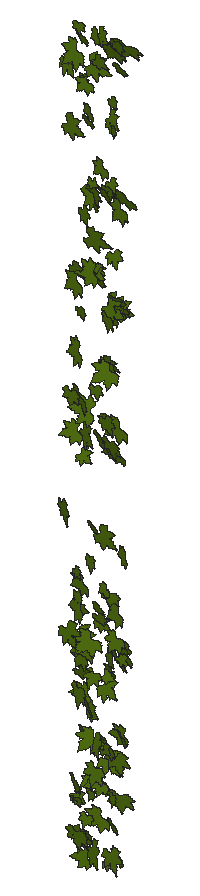
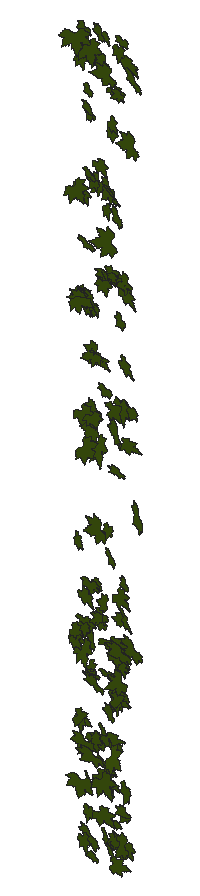
# SketchUp Ruby script. Lengths in inches.
U = 1.inch
M = Sketchup.active_model
def pt(a) = Geom::Point3d.new(a.map { |v| v * U })
def face(e, loops, mat)
  f = e.add_face(loops[0].map { |a| pt(a) })
  loops[1..].each { |l| e.add_face(l.map { |a| pt(a) }).erase! }
  f.material = f.back_material = mat if mat
  f
end
# faces: each face lists its corners as indices into pts; further lists are holes
def faces(e, pts, list, mat = nil) = list.each { |f| face(e, (f[0].is_a?(Array) ? f : [f]).map { |l| l.map { |i| pts[i] } }, mat) }
# xy, xz, yz: faces in a plane at the given z, y or x. An outline is a flat list of corners, or four numbers for a rectangle; further outlines are holes
def ring(l) = l.size == 4 ? [[l[0], l[1]], [l[2], l[1]], [l[2], l[3]], [l[0], l[3]]] : l.each_slice(2).to_a
def flat(e, list, mat, &to3) = list.each { |f| face(e, (f[0].is_a?(Array) ? f : [f]).map { |l| ring(l).map { |u, v| to3.(u, v) } }, mat) }
def xy(e, z, list, mat = nil) = flat(e, list, mat) { |x, y| [x, y, z] }
def xz(e, y, list, mat = nil) = flat(e, list, mat) { |x, z| [x, y, z] }
def yz(e, x, list, mat = nil) = flat(e, list, mat) { |y, z| [x, y, z] }
def lines(e, pts, list) = list.each { |a, b| e.add_line(pt(pts[a]), pt(pts[b])) }
# prism: a flat outline (further loops are holes) pulled along v
def prism(e, loops, v, mat = nil)
  f = face(e, loops, mat); d = Geom::Vector3d.new(v.map { |x| x * U })
  f.pushpull(f.normal.samedirection?(d) ? d.length : -d.length)
end
def box(e, o, s, mat = nil) = prism(e, [[o, [o[0] + s[0], o[1], o[2]], [o[0] + s[0], o[1] + s[1], o[2]], [o[0], o[1] + s[1], o[2]]]], [0, 0, s[2]], mat)
def at(x, y, z, deg = 0) = Geom::Transformation.translation(pt([x, y, z])) * Geom::Transformation.rotation(ORIGIN, Z_AXIS, deg.degrees)
def axes(o, x, y, z) = Geom::Transformation.new([*x, 0, *y, 0, *z, 0, *pt(o).to_a, 1])
def part(name) = M.definitions.add(name)
# library, detail: a bought-in or finely detailed component or shape, given as its bounding box
def library(name, o, s) = part(name).tap { |d| box(d.entities, o, s) }
def detail(e, o, s) = box(e.add_group.entities, o, s)
def put(e, d, t, mat = nil) = e.add_instance(d, t).tap { |i| i.material = mat if mat }
def group(e, t, mat = nil) = e.add_group.tap { |g| g.transformation = t; g.material = mat if mat }.entities
root = M.entities
M.materials.add("[Vegetation Blur 03]").color = [83, 114, 18]
c1 = part("ivy")
xy(c1.entities,0,[[0.782,0,0.786,0,0.787,0.005,0.789,0.009,0.821,0.072,0.875,0.147,1.001,0.272,1.073,0.331,1.137,0.363,1.178,0.379,1.223,0.384,1.272,0.383,1.311,0.374,1.36,0.355,1.399,0.334,1.491,0.285,1.541,0.244,1.583,0.199,1.617,0.15,1.64,0.128,1.662,0.115,1.717,0.105,1.745,0.093,1.784,0.054,1.819,0.057,1.854,0.064,1.882,0.075,1.896,0.074,1.91,0.071,1.937,0.063,1.964,0.053,1.99,0.038,2.016,0.015,2.034,0.002,2.04,0,2.038,0.003,2.036,0.007,2.033,0.038,2.036,0.068,2.045,0.1,2.055,0.116,2.064,0.123,2.077,0.129,2.088,0.129,2.106,0.132,2.118,0.13,2.179,0.132,2.207,0.133,2.225,0.133,2.242,0.138,2.22,0.162,2.207,0.186,2.206,0.213,2.212,0.236,2.228,0.262,2.247,0.274,2.298,0.283,2.355,0.294,2.37,0.296,2.376,0.295,2.377,0.3,2.377,0.303,2.385,0.329,2.411,0.37,2.426,0.392,2.449,0.407,2.511,0.426,2.561,0.444,2.619,0.466,2.589,0.469,2.561,0.476,2.501,0.5,2.449,0.516,2.424,0.523,2.401,0.535,2.377,0.556,2.372,0.568,2.36,0.575,2.268,0.586,2.225,0.592,2.207,0.599,2.194,0.61,2.143,0.65,2.13,0.664,2.122,0.682,2.123,0.7,2.13,0.719,2.148,0.75,2.17,0.781,2.195,0.807,2.221,0.828,2.284,0.874,2.291,0.88,2.288,0.887,2.276,0.9,2.267,0.916,2.265,0.933,2.273,0.967,2.292,1.002,2.313,1.03,2.334,1.054,2.348,1.067,2.358,1.074,2.363,1.076,2.362,1.081,2.35,1.094,2.347,1.11,2.35,1.143,2.359,1.18,2.385,1.254,2.415,1.324,2.448,1.393,2.45,1.4,2.446,1.398,2.44,1.394,2.427,1.383,2.402,1.36,2.376,1.339,2.345,1.324,2.305,1.309,2.282,1.303,2.273,1.306,2.245,1.294,2.212,1.287,2.187,1.291,2.163,1.301,2.142,1.316,2.134,1.327,2.124,1.325,2.09,1.292,2.053,1.259,2.014,1.234,1.973,1.215,1.954,1.21,1.931,1.208,1.909,1.212,1.893,1.22,1.879,1.233,1.872,1.248,1.867,1.281,1.864,1.319,1.821,1.258,1.773,1.197,1.726,1.141,1.698,1.121,1.679,1.116,1.666,1.117,1.647,1.122,1.632,1.129,1.62,1.141,1.617,1.154,1.617,1.219,1.621,1.254,1.623,1.268,1.623,1.281,1.618,1.314,1.606,1.346,1.603,1.375,1.607,1.403,1.603,1.467,1.599,1.499,1.605,1.525,1.614,1.552,1.629,1.577,1.635,1.589,1.629,1.587,1.618,1.582,1.596,1.566,1.581,1.556,1.568,1.552,1.557,1.55,1.545,1.553,1.531,1.562,1.522,1.572,1.504,1.591,1.486,1.611,1.474,1.631,1.457,1.666,1.455,1.684,1.457,1.698,1.452,1.715,1.444,1.728,1.424,1.754,1.419,1.772,1.423,1.786,1.434,1.819,1.444,1.848,1.446,1.855,1.44,1.861,1.43,1.867,1.386,1.904,1.349,1.948,1.326,1.973,1.31,1.995,1.288,2.048,1.284,2.153,1.287,2.254,1.284,2.255,1.282,2.253,1.278,2.247,1.274,2.237,1.266,2.216,1.226,2.125,1.208,2.076,1.184,2.033,1.155,1.984,1.135,1.942,1.111,1.899,1.083,1.861,1.053,1.85,1.059,1.83,1.061,1.809,1.056,1.79,1.049,1.767,1.04,1.749,1.018,1.733,0.994,1.726,0.942,1.734,0.95,1.6875,0.944,1.645,0.932,1.608,0.911,1.585,0.881,1.58,0.854,1.582,0.828,1.588,0.785,1.618,0.773,1.625,0.775,1.614,0.779,1.598,0.796,1.502,0.818,1.402,0.861,1.283,0.882,1.224,0.894,1.174,0.892,1.148,0.886,1.123,0.881,1.107,0.872,1.099,0.849,1.094,0.818,1.092,0.789,1.098,0.762,1.107,0.753,1.113,0.721,1.139,0.698,1.163,0.678,1.194,0.665,1.224,0.628,1.28,0.612,1.312,0.606,1.327,0.606,1.314,0.599,1.282,0.594,1.267,0.581,1.256,0.544,1.245,0.512,1.244,0.473,1.249,0.444,1.256,0.382,1.288,0.339,1.306,0.324,1.316,0.317,1.324,0.309,1.326,0.27,1.314,0.227,1.313,0.185,1.3125,0.152,1.317,0.122,1.328,0.092,1.345,0.073,1.353,0.079,1.338,0.092,1.308,0.117,1.249,0.13,1.215,0.139,1.164,0.147,1.148,0.157,1.136,0.163,1.122,0.174,1.086,0.177,1.067,0.182,1.054,0.186,1.043,0.191,1.038,0.211,1.028,0.237,1.005,0.25,0.974,0.253,0.96,0.25,0.944,0.242,0.914,0.243,0.906,0.249,0.902,0.26,0.894,0.289,0.88,0.307,0.873,0.322,0.862,0.364,0.799,0.403,0.738,0.431,0.709,0.439,0.691,0.441,0.678,0.4375,0.66,0.428,0.645,0.394,0.623,0.303,0.594,0.255,0.581,0.214,0.577,0.179,0.573,0.173,0.568,0.175,0.561,0.167,0.55,0.141,0.523,0.113,0.503,0.077,0.49,0.045,0.486,0.026,0.485,0.019,0.486,0.011,0.483,0,0.471,0.014,0.467,0.044,0.455,0.058,0.447,0.07,0.438,0.097,0.411,0.125,0.394,0.158,0.377,0.174,0.366,0.182,0.359,0.185,0.361,0.242,0.331,0.253,0.316,0.258,0.303,0.262,0.283,0.274,0.278,0.308,0.274,0.341,0.252,0.366,0.226,0.366,0.222,0.37,0.22,0.38,0.221,0.395,0.221,0.425,0.216,0.45,0.207,0.465,0.192,0.473,0.178,0.484,0.15,0.489,0.116,0.483,0.089,0.468,0.058,0.45,0.035,0.435,0.018,0.429,0.011,0.434,0.012,0.438,0.014,0.469,0.019,0.542,0.016,0.581,0.015,0.612,0.027,0.68,0.055,0.696,0.057,0.712,0.052,0.73,0.045,0.741,0.036,0.766,0.014]])
put(root,c1,axes([70.27,173.7,76.7],[0.25465,-0.11048,-0.36792],[-0.45313,-0.12762,-0.20287],[0.02807,-1.05778,0.0629]),"[Vegetation Blur 03]")
put(root,c1,axes([69.17,173.7,94.66],[0.3032,0.00804,0.42723],[0.50376,-0.343,-0.23711],[-0.14236,-1.19666,0.07083]),"[Vegetation Blur 03]")
put(root,c1,axes([69.13,173.7,72.18],[0.48124,-0.36893,0.30519],[0.35516,-0.24188,-0.41903],[-0.21409,-1.23057,-0.00913]),"[Vegetation Blur 03]")
put(root,c1,axes([69.06,173.7,65.4375],[0.45366,-0.05419,0.38117],[0.46073,-0.18,-0.36926],[-0.08098,-1.3277,0.0345]),"[Vegetation Blur 03]")
put(root,c1,axes([69.46,173.7,78.17],[0.49069,-0.15556,0.05335],[0.06086,-0.06942,-0.40473],[-0.07927,-1.0163,0.01948]),"[Vegetation Blur 03]")
put(root,c1,axes([70.36,173.7,80.93],[0.29092,-0.24551,-0.40873],[-0.49509,0.19114,-0.25278],[-0.14116,-1.1764,0.04423]),"[Vegetation Blur 03]")
put(root,c1,axes([70.1,173.7,84.52],[0.43677,-0.25618,-0.34823],[-0.42807,0.08886,-0.36791],[-0.11962,-1.25334,0.04509]),"[Vegetation Blur 03]")
put(root,c1,axes([70.52,173.7,67.91],[0.26701,-0.30376,-0.4486],[-0.53833,0.27065,-0.24226],[-0.1847,-1.22801,0.05757]),"[Vegetation Blur 03]")
put(root,c1,axes([69.35,173.7,91.19],[0.18628,-0.03587,0.49266],[0.60208,-0.08964,-0.15266],[-0.04677,-1.29689,-0.00307]),"[Vegetation Blur 03]")
put(root,c1,axes([70.78,173.7,60.76],[0.09506,0.21771,-0.46057],[-0.55663,0.32363,-0.05246],[-0.14082,-1.13231,-0.10355]),"[Vegetation Blur 03]")
put(root,c1,axes([70.41,173.7,68.89],[0.30205,-0.06223,-0.36549],[-0.44449,0.11303,-0.2477],[-0.06243,-1.1058,-0.00475]),"[Vegetation Blur 03]")
put(root,c1,axes([69.84,173.7,57.14],[0.28399,-0.06546,0.07539],[0.09562,0.06624,-0.23087],[-0.02006,-0.61097,-0.03311]),"[Vegetation Blur 03]")
put(root,c1,axes([70.01,173.7,96.4],[0.54958,-0.28156,-0.28314],[-0.3622,-0.10008,-0.45262],[-0.08884,-1.33367,0.09374]),"[Vegetation Blur 03]")
put(root,c1,axes([69.77,173.7,57.02],[0.18546,0.05213,0.26962],[0.33131,-0.03649,-0.15069],[-0.00311,-0.77875,0.02511]),"[Vegetation Blur 03]")
put(root,c1,axes([69.85,173.7,58.47],[0.46353,-0.32199,-0.04056],[-0.03174,0.12476,-0.39742],[-0.16108,-0.95117,-0.0384]),"[Vegetation Blur 03]")
put(root,c1,axes([69.72,173.7,84.26],[0.26264,-0.10696,0.28896],[0.35555,-0.0243,-0.21667],[-0.0405,-0.90682,-0.02828]),"[Vegetation Blur 03]")
put(root,c1,axes([69.58,173.7,55.66],[0.62439,-0.15847,0.04406],[0.05688,0.04229,-0.51297],[-0.0749,-1.28898,-0.02225]),"[Vegetation Blur 03]")
put(root,c1,axes([70,173.7,97.09],[0.3174,-0.05029,0.04385],[0.05287,-0.02687,-0.25971],[-0.02626,-0.66189,0.00721]),"[Vegetation Blur 03]")
put(root,c1,axes([69.97,173.7,68.77],[0.18692,-0.08145,0.20202],[0.24238,-0.1034,-0.15594],[-0.06396,-0.62987,-0.00053]),"[Vegetation Blur 03]")
put(root,c1,axes([70.09,173.7,78.54],[0.55558,-0.31709,-0.23093],[-0.26347,0.22092,-0.46992],[-0.18545,-1.26384,-0.0242]),"[Vegetation Blur 03]")
put(root,c1,axes([70.9375,173.7,63.32],[0.10909,-0.05884,-0.38294],[-0.46937,-0.06819,-0.08742],[0.02587,-0.98895,0.02881]),"[Vegetation Blur 03]")
put(root,c1,axes([71.01,173.7,54.81],[0.07011,-0.04175,-0.39035],[-0.47768,-0.07166,-0.05594],[0.03155,-0.99215,0.02047]),"[Vegetation Blur 03]")
put(root,c1,axes([70.23,173.7,96.76],[0.35771,-0.12648,-0.10441],[-0.11497,0.1604,-0.29291],[-0.08323,-0.76513,-0.04414]),"[Vegetation Blur 03]")
put(root,c1,axes([70.19,173.7,65.06],[0.4568,-0.18649,-0.14633],[-0.18134,0.01163,-0.3794],[-0.08646,-1.00976,0.02265]),"[Vegetation Blur 03]")
put(root,c1,axes([70.73,173.7,65.83],[0.34831,-0.13161,-0.42418],[-0.52189,0.01831,-0.28634],[-0.04303,-1.28736,0.03929]),"[Vegetation Blur 03]")
put(root,c1,axes([70.09,173.7,74.53],[0.15249,0.14355,0.27563],[0.34484,-0.05498,-0.12257],[0.00385,-0.76056,0.06089]),"[Vegetation Blur 03]")
put(root,c1,axes([69.67,173.7,65.11],[0.33086,0.13392,0.42114],[0.51995,-0.11554,-0.26631],[-0.01255,-1.25609,0.0694]),"[Vegetation Blur 03]")
put(root,c1,axes([70.1875,173.7,94.08],[0.20167,-0.04503,0.17751],[0.21848,0.0617,-0.16287],[0.00725,-0.60725,-0.02971]),"[Vegetation Blur 03]")
put(root,c1,axes([70.33,173.7,66.78],[0.04043,-0.04833,0.23762],[0.29161,-0.02839,-0.03396],[-0.01694,-0.60422,-0.01741]),"[Vegetation Blur 03]")
put(root,c1,axes([70.14,173.7,82.4],[0.29752,-0.1463,0.14185],[0.17418,-0.03541,-0.24908],[-0.07018,-0.70816,-0.01685]),"[Vegetation Blur 03]")
put(root,c1,axes([69.99,173.7,54.9],[0.12855,-0.09811,0.43066],[0.52964,-0.00555,-0.1055],[-0.01392,-1.1176,-0.03728]),"[Vegetation Blur 03]")
put(root,c1,axes([70.92,173.7,93.07],[0.17412,-0.05091,-0.27988],[-0.33267,0.17495,-0.14285],[-0.08689,-0.77186,-0.01392]),"[Vegetation Blur 03]")
put(root,c1,axes([71.375,173.7,78.18],[0.08303,-0.1967,-0.5076],[-0.62878,-0.07669,-0.06383],[0.02474,-1.28895,0.08126]),"[Vegetation Blur 03]")
put(root,c1,axes([70.59,173.7,94.65],[0.37323,-0.08724,-0.21133],[-0.2619,-0.06711,-0.30372],[-0.01607,-0.93236,0.04164]),"[Vegetation Blur 03]")
put(root,c1,axes([69.97,173.7,63.18],[0.5531,-0.30937,0.07702],[0.082,-0.11827,-0.46698],[-0.15743,-1.14854,0.02734]),"[Vegetation Blur 03]")
put(root,c1,axes([69.96,173.7,63.6],[0.33482,-0.12296,0.29954],[0.37174,0.13576,-0.26801],[0.00918,-1.01326,-0.07226]),"[Vegetation Blur 03]")
put(root,c1,axes([70.625,173.7,92.47],[0.29211,-0.05666,-0.12031],[-0.1385,0.15286,-0.23529],[-0.05752,-0.65573,-0.04445]),"[Vegetation Blur 03]")
put(root,c1,axes([70.9375,173.7,58.68],[0.22279,-0.12525,-0.19809],[-0.24846,-0.03124,-0.18302],[-0.02974,-0.67725,0.04508]),"[Vegetation Blur 03]")
put(root,c1,axes([70.52,173.7,56.61],[0.33968,-0.06301,-0.00772],[-0.01455,-0.11855,-0.2742],[-0.02856,-0.68915,0.04788]),"[Vegetation Blur 03]")
put(root,c1,axes([71.28,173.7,85.27],[0.22309,-0.1604,-0.43567],[-0.53899,-0.01598,-0.18291],[-0.02282,-1.19045,0.06116]),"[Vegetation Blur 03]")
put(root,c1,axes([70.65,173.7,66.2],[0.52837,-0.04737,-0.26503],[-0.32337,-0.22367,-0.42312],[0.03764,-1.25647,0.08531]),"[Vegetation Blur 03]")
put(root,c1,axes([71.47,173.7,89.38],[0.14321,-0.30149,-0.44399],[-0.54717,0.20081,-0.13901],[-0.13425,-1.14006,0.09293]),"[Vegetation Blur 03]")
put(root,c1,axes([70.48,173.7,55.37],[0.20518,-0.11933,0.20995],[0.26085,-0.0065,-0.17038],[-0.03866,-0.67709,-0.03537]),"[Vegetation Blur 03]")
put(root,c1,axes([70.3,173.7,87.49],[0.34266,-0.16677,0.2483],[0.29126,-0.18349,-0.28712],[-0.11956,-0.92493,0.01219]),"[Vegetation Blur 03]")
put(root,c1,axes([70.83,173.7,61.21],[0.5099,-0.05447,-0.26558],[-0.32487,-0.20771,-0.40876],[0.03235,-1.22728,0.08097]),"[Vegetation Blur 03]")
put(root,c1,axes([71.1,173.7,88.44],[0.23798,-0.09799,-0.20106],[-0.2294,0.19812,-0.19604],[-0.10166,-0.67644,-0.02829]),"[Vegetation Blur 03]")
put(root,c1,axes([71.13,173.7,59.16],[0.44315,0.00145,-0.39097],[-0.47521,0.17095,-0.35867],[-0.06051,-1.33197,-0.04646]),"[Vegetation Blur 03]")
put(root,c1,axes([70.87,173.7,71.7],[0.31001,-0.14403,-0.03677],[-0.03088,0.13304,-0.25536],[-0.0773,-0.63077,-0.04546]),"[Vegetation Blur 03]")
put(root,c1,axes([71.07,173.7,84.65],[0.35037,-0.01321,-0.20166],[-0.24181,0.16441,-0.28153],[-0.0512,-0.86678,-0.05033]),"[Vegetation Blur 03]")
put(root,c1,axes([70.59,173.7,84.83],[0.4392,0.07424,0.06802],[0.08567,-0.05755,-0.35857],[0.03015,-0.91812,0.02798]),"[Vegetation Blur 03]")
put(root,c1,axes([70.9375,173.7,58.1],[0.29646,-0.18293,-0.03481],[-0.04858,-0.02904,-0.25162],[-0.08579,-0.61566,0.02221]),"[Vegetation Blur 03]")
put(root,c1,axes([70.31,173.7,62.93],[0.62192,-0.51222,0.08279],[0.13225,0.12501,-0.54004],[-0.23401,-1.29066,-0.08517]),"[Vegetation Blur 03]")
put(root,c1,axes([70.38,173.7,75.84],[0.18528,-0.05644,0.53215],[0.61865,-0.42892,-0.15063],[-0.2078,-1.32731,0.02605]),"[Vegetation Blur 03]")
put(root,c1,axes([70.78,173.7,61.59],[0.06873,0.01711,0.34805],[0.41669,-0.19262,-0.05332],[-0.09114,-0.86777,0.0187]),"[Vegetation Blur 03]")
put(root,c1,axes([70.87,173.7,64.16],[0.41492,-0.08686,-0.03354],[-0.04844,-0.1605,-0.33372],[-0.03354,-0.84286,0.067]),"[Vegetation Blur 03]")
put(root,c1,axes([71.35,173.7,97.22],[0.22954,-0.17233,-0.19599],[-0.23774,0.09106,-0.19805],[-0.09034,-0.67751,0.02323]),"[Vegetation Blur 03]")
put(root,c1,axes([70.76,173.7,69.9],[0.3651,-0.20886,0.13721],[0.15459,-0.14475,-0.30864],[-0.12111,-0.81437,0.01967]),"[Vegetation Blur 03]")
put(root,c1,axes([71.375,173.7,57.28],[0.4097,-0.04709,-0.34938],[-0.42867,-0.05903,-0.33358],[0.00494,-1.21793,0.02968]),"[Vegetation Blur 03]")
put(root,c1,axes([71.34,173.7,76.47],[0.46716,-0.062,-0.38996],[-0.44887,0.42109,-0.3687],[-0.16652,-1.30905,-0.10013]),"[Vegetation Blur 03]")
put(root,c1,axes([70.61,173.7,94.5],[0.13182,0.09274,0.49871],[0.61259,0.00582,-0.10802],[0.01227,-1.28635,0.03547]),"[Vegetation Blur 03]")
put(root,c1,axes([70.9,173.7,84.14],[0.09631,0.08819,0.32844],[0.40359,-0.08421,-0.07527],[-0.03009,-0.84734,0.04167]),"[Vegetation Blur 03]")
put(root,c1,axes([71.58,173.7,59.16],[0.31711,-0.08877,-0.37028],[-0.45541,-0.10498,-0.25583],[0.01733,-1.13422,0.05266]),"[Vegetation Blur 03]")
put(root,c1,axes([70.91,173.7,78.63],[0.33984,-0.05336,0.11192],[0.13528,-0.05673,-0.27786],[-0.03432,-0.75199,0.01302]),"[Vegetation Blur 03]")
put(root,c1,axes([70.62,173.7,85.74],[0.17934,-0.09894,0.51265],[0.6295,0.08025,-0.14425],[0.02442,-1.34184,-0.04643]),"[Vegetation Blur 03]")
put(root,c1,axes([70.7,173.7,88.88],[0.47833,-0.24749,0.17674],[0.22101,-0.01127,-0.40089],[-0.11188,-1.08043,-0.0363]),"[Vegetation Blur 03]")
put(root,c1,axes([70.87,173.7,59.41],[0.56213,-0.17838,-0.00831],[-0.02255,-0.16495,-0.45927],[-0.08432,-1.14512,0.06745]),"[Vegetation Blur 03]")
put(root,c1,axes([71.54,173.7,90.62],[0.34594,-0.11487,-0.25725],[-0.31497,0.04827,-0.28551],[-0.05712,-0.96184,0.01639]),"[Vegetation Blur 03]")
put(root,c1,axes([71.07,173.7,66.89],[0.3213,-0.06644,0.14929],[0.18483,0.03966,-0.26218],[-0.01845,-0.75978,-0.02674]),"[Vegetation Blur 03]")
put(root,c1,axes([71.07,173.7,95.24],[0.18668,-0.06069,0.28857],[0.35478,0.02187,-0.15215],[-0.00434,-0.8225,-0.02534]),"[Vegetation Blur 03]")
put(root,c1,axes([71.27,173.7,67.22],[0.06463,-0.12992,0.26421],[0.32679,-0.06667,-0.0584],[-0.04465,-0.67604,-0.04502]),"[Vegetation Blur 03]")
put(root,c1,axes([70.9,173.7,60.37],[0.33688,-0.08622,0.33874],[0.38873,-0.33347,-0.27086],[-0.15137,-1.04826,0.0583]),"[Vegetation Blur 03]")
put(root,c1,axes([70.83,173.7,54.63],[0.29467,-0.10714,0.44848],[0.50944,-0.44068,-0.23951],[-0.21249,-1.20507,0.04772]),"[Vegetation Blur 03]")
put(root,c1,axes([71.14,173.7,66.36],[0.19136,0.01715,0.31471],[0.38568,-0.01715,-0.15606],[-0.00376,-0.88569,0.00911]),"[Vegetation Blur 03]")
put(root,c1,axes([71.7,173.7,77.49],[0.29858,0.09929,-0.17499],[-0.21887,0.06675,-0.24279],[0.01995,-0.75348,-0.04457]),"[Vegetation Blur 03]")
put(root,c1,axes([71.84,173.7,68.86],[0.2154,-0.10325,-0.19292],[-0.23671,0.04089,-0.17948],[-0.04859,-0.65681,0.01915]),"[Vegetation Blur 03]")
put(root,c1,axes([72.08,173.7,64.61],[0.12889,0.05373,-0.25764],[-0.31029,0.16238,-0.09807],[-0.06367,-0.68262,-0.04361]),"[Vegetation Blur 03]")
put(root,c1,axes([71.71,173.7,60.93],[0.42245,-0.13873,-0.23601],[-0.28027,0.15555,-0.34853],[-0.09809,-1.04193,-0.02061]),"[Vegetation Blur 03]")
put(root,c1,axes([71.35,173.7,96.58],[0.1212,0.00874,0.32904],[0.39357,-0.19062,-0.09576],[-0.08752,-0.84508,0.025]),"[Vegetation Blur 03]")
put(root,c1,axes([71.56,173.7,63.65],[0.07011,0.12287,0.23012],[0.28735,0.0166,-0.05971],[0.0224,-0.59768,0.04565]),"[Vegetation Blur 03]")
put(root,c1,axes([71.27,173.7,60.1],[0.22931,-0.05412,0.29769],[0.36487,-0.02596,-0.18795],[-0.02469,-0.88622,-0.01267]),"[Vegetation Blur 03]")
put(root,c1,axes([72.39,173.7,76.09],[0.19085,0.16255,-0.44019],[-0.54494,0.0863,-0.15236],[-0.01363,-1.17416,-0.07214]),"[Vegetation Blur 03]")
put(root,c1,axes([71.71,173.7,96.74],[0.51903,0.05216,-0.26245],[-0.32095,0.20906,-0.41624],[-0.03231,-1.23893,-0.08129]),"[Vegetation Blur 03]")
put(root,c1,axes([71.91,173.7,80.56],[0.49181,-0.15671,-0.3315],[-0.41314,-0.21702,-0.39213],[0.00973,-1.29451,0.10587]),"[Vegetation Blur 03]")
put(root,c1,axes([71.67,173.7,54.15],[0.08845,0.08211,0.23234],[0.28731,-0.04554,-0.07032],[-0.00952,-0.61175,0.03642]),"[Vegetation Blur 03]")
put(root,c1,axes([71.4,173.7,89.0625],[0.39765,-0.2594,0.13842],[0.18466,0.06494,-0.33421],[-0.10274,-0.88724,-0.06493]),"[Vegetation Blur 03]")
put(root,c1,axes([71.11,173.7,70.82],[0.30964,-0.0676,0.45983],[0.56279,-0.06237,-0.25387],[-0.0424,-1.3215,-0.01154]),"[Vegetation Blur 03]")
put(root,c1,axes([71.28,173.7,62.93],[0.19869,0.16598,0.44202],[0.5434,-0.20587,-0.15053],[-0.06748,-1.16914,0.08926]),"[Vegetation Blur 03]")
put(root,c1,axes([71.625,173.7,89.17],[0.34101,-0.13421,0.11002],[0.1371,0.00224,-0.28262],[-0.06025,-0.75456,-0.02041]),"[Vegetation Blur 03]")
put(root,c1,axes([71.26,173.7,59.34],[0.3778,0.16016,0.36511],[0.45377,-0.08873,-0.30663],[0.01685,-1.20168,0.0713]),"[Vegetation Blur 03]")
put(root,c1,axes([72.4375,173.7,83.13],[0.17466,-0.11177,-0.29584],[-0.34642,0.21964,-0.14928],[-0.11976,-0.79834,0.00035]),"[Vegetation Blur 03]")
put(root,c1,axes([71.45,173.7,80],[0.29936,-0.14494,0.31849],[0.3965,0.0953,-0.24142],[-0.00556,-1.00761,-0.06865]),"[Vegetation Blur 03]")
put(root,c1,axes([72.23,173.7,65.64],[0.40831,-0.04926,-0.36189],[-0.41615,0.39004,-0.3211],[-0.15494,-1.17746,-0.09123]),"[Vegetation Blur 03]")
put(root,c1,axes([71.72,173.7,68.53],[0.44619,-0.06474,-0.00167],[-0.00306,-0.02944,-0.36486],[-0.03138,-0.91771,0.01182]),"[Vegetation Blur 03]")
put(root,c1,axes([71.44,173.7,77.14],[0.40671,-0.14437,0.24599],[0.29835,-0.08915,-0.33679],[-0.0822,-1.03788,-0.00529]),"[Vegetation Blur 03]")
put(root,c1,axes([71.68,173.7,82.79],[0.45964,-0.254,0.03008],[0.03689,-0.00973,-0.3884],[-0.12342,-0.94883,-0.00407]),"[Vegetation Blur 03]")
put(root,c1,axes([72.86,173.7,83.72],[0.10531,0.2061,-0.4524],[-0.56328,0.04564,-0.08406],[-0.00345,-1.16018,-0.08367]),"[Vegetation Blur 03]")
put(root,c1,axes([72.03,173.7,56.83],[0.35108,-0.18402,-0.07774],[-0.07773,0.15757,-0.29247],[-0.10502,-0.7318,-0.04343]),"[Vegetation Blur 03]")
put(root,c1,axes([72.41,173.7,77.68],[0.41789,-0.06408,-0.38347],[-0.47,0.02266,-0.34176],[-0.02893,-1.29377,0.01301]),"[Vegetation Blur 03]")
put(root,c1,axes([71.96,173.7,79.7],[0.0683,-0.05119,0.27634],[0.33407,-0.11649,-0.05839],[-0.06049,-0.70118,-0.01047]),"[Vegetation Blur 03]")
put(root,c1,axes([71.85,173.7,89.29],[0.21707,0.00977,0.22202],[0.26718,-0.14285,-0.17301],[-0.05136,-0.70178,0.03831]),"[Vegetation Blur 03]")
put(root,c1,axes([71.5625,173.7,82.47],[0.16468,0.13945,0.51477],[0.63081,-0.17776,-0.12684],[-0.06707,-1.32961,0.07095]),"[Vegetation Blur 03]")
put(root,c1,axes([71.84,173.7,92.37],[0.13518,0.07282,0.36034],[0.43243,-0.22734,-0.10083],[-0.09589,-0.9226,0.05329]),"[Vegetation Blur 03]")
put(root,c1,axes([72,173.7,93.61],[0.18338,-0.0476,0.19783],[0.23906,-0.08339,-0.15076],[-0.04624,-0.61987,0.00509]),"[Vegetation Blur 03]")
put(root,c1,axes([72.49,173.7,68.17],[0.36665,-0.19895,-0.32997],[-0.4044,0.08632,-0.30749],[-0.09631,-1.11984,0.03492]),"[Vegetation Blur 03]")
put(root,c1,axes([72.36,173.7,55.47],[0.35757,-0.14861,-0.22341],[-0.2596,0.18993,-0.29662],[-0.11295,-0.907,-0.02551]),"[Vegetation Blur 03]")
put(root,c1,axes([72.26,173.7,66.33],[0.32932,-0.07979,-0.11263],[-0.13041,0.12861,-0.26832],[-0.05951,-0.72344,-0.03528]),"[Vegetation Blur 03]")
put(root,c1,axes([71.625,173.7,76.36],[0.58972,-0.25941,0.10506],[0.13617,0.04808,-0.49046],[-0.11798,-1.24117,-0.04096]),"[Vegetation Blur 03]")
put(root,c1,axes([71.92,173.7,64.97],[0.15407,-0.1087,0.33806],[0.39127,-0.27976,-0.13293],[-0.14585,-0.86534,0.00051]),"[Vegetation Blur 03]")
put(root,c1,axes([72.47,173.7,95.77],[0.26625,0.02526,-0.1848],[-0.22371,0.14694,-0.21152],[-0.03714,-0.70407,-0.05077]),"[Vegetation Blur 03]")
put(root,c1,axes([72.95,173.7,61.84],[0.13243,-0.0083,-0.40164],[-0.49158,0.04791,-0.10811],[-0.02353,-1.04762,-0.00176]),"[Vegetation Blur 03]")
put(root,c1,axes([72.04,173.7,92.57],[0.32682,-0.209,0.08086],[0.0994,-0.02803,-0.27901],[-0.10124,-0.70219,-0.01293]),"[Vegetation Blur 03]")
put(root,c1,axes([71.89,173.7,85.73],[0.33502,0.02499,0.20079],[0.2423,-0.1873,-0.26561],[-0.04435,-0.83458,0.06562]),"[Vegetation Blur 03]")
put(root,c1,axes([72.86,173.7,83.3125],[0.07838,0.01913,-0.25028],[-0.30675,-0.00782,-0.06408],[0.00599,-0.6513,-0.00658]),"[Vegetation Blur 03]")
put(root,c1,axes([72.68,173.7,89.28],[0.33022,0.14446,-0.3444],[-0.42741,0.15711,-0.26261],[-0.01782,-1.09139,-0.08339]),"[Vegetation Blur 03]")
put(root,c1,axes([72.18,173.7,58.15],[0.27567,-0.18278,0.07916],[0.08,-0.13493,-0.23455],[-0.1044,-0.58604,0.02931]),"[Vegetation Blur 03]")
put(root,c1,axes([72.17,173.7,66.61],[0.48596,-0.138,-0.11802],[-0.15256,-0.12597,-0.39525],[-0.04619,-1.03571,0.0638]),"[Vegetation Blur 03]")
put(root,c1,axes([71.63,173.7,54.98],[0.51611,-0.14167,0.29822],[0.35265,-0.22138,-0.42305],[-0.1179,-1.28232,0.04009]),"[Vegetation Blur 03]")
put(root,c1,axes([72.32,173.7,83.2],[0.33133,0.03179,-0.00697],[-0.01113,0.11989,-0.26643],[0.0137,-0.67142,-0.0479]),"[Vegetation Blur 03]")
put(root,c1,axes([73,173.7,70.95],[0.13696,-0.09293,-0.32969],[-0.38837,0.22901,-0.11762],[-0.11998,-0.84735,0.00437]),"[Vegetation Blur 03]")
put(root,c1,axes([72.53,173.7,61.54],[0.33215,-0.12492,-0.16924],[-0.19211,0.18741,-0.2729],[-0.09889,-0.78367,-0.03828]),"[Vegetation Blur 03]")
put(root,c1,axes([72.1,173.7,96.86],[0.38814,-0.14356,0.10109],[0.12917,0.04667,-0.31993],[-0.05936,-0.83711,-0.03517]),"[Vegetation Blur 03]")
put(root,c1,axes([71.92,173.7,58.25],[0.6157,0.01002,0.02515],[0.03061,0.04996,-0.50212],[0.00607,-1.26758,-0.01959]),"[Vegetation Blur 03]")
put(root,c1,axes([71.77,173.7,60.03],[0.55674,-0.05035,0.19483],[0.23814,-0.03752,-0.45478],[-0.02967,-1.24598,0.00582]),"[Vegetation Blur 03]")
put(root,c1,axes([72.26,173.7,97.05],[0.59461,0.12109,-0.18026],[-0.22736,0.18289,-0.48022],[0.02354,-1.29241,-0.08484]),"[Vegetation Blur 03]")
put(root,c1,axes([72.11,173.7,82.58],[0.10294,0.13872,0.40661],[0.50198,0.02961,-0.08624],[0.02785,-1.04645,0.05146]),"[Vegetation Blur 03]")
put(root,c1,axes([72.48,173.7,88.94],[0.49987,-0.22483,-0.22694],[-0.27931,0.04426,-0.41667],[-0.10606,-1.17624,0.0277]),"[Vegetation Blur 03]")
put(root,c1,axes([73.13,173.7,65.54],[0.04662,-0.02211,-0.24119],[-0.29524,-0.03871,-0.03745],[0.01692,-0.61444,0.01104]),"[Vegetation Blur 03]")
put(root,c1,axes([73.04,173.7,65.9],[0.21141,-0.03642,-0.34067],[-0.40654,0.204,-0.17147],[-0.09632,-0.94099,-0.02399]),"[Vegetation Blur 03]")
put(root,c1,axes([73.14,173.7,66.15],[0.07372,0.06524,-0.26494],[-0.3259,0.04312,-0.05873],[-0.01352,-0.68368,-0.02899]),"[Vegetation Blur 03]")
